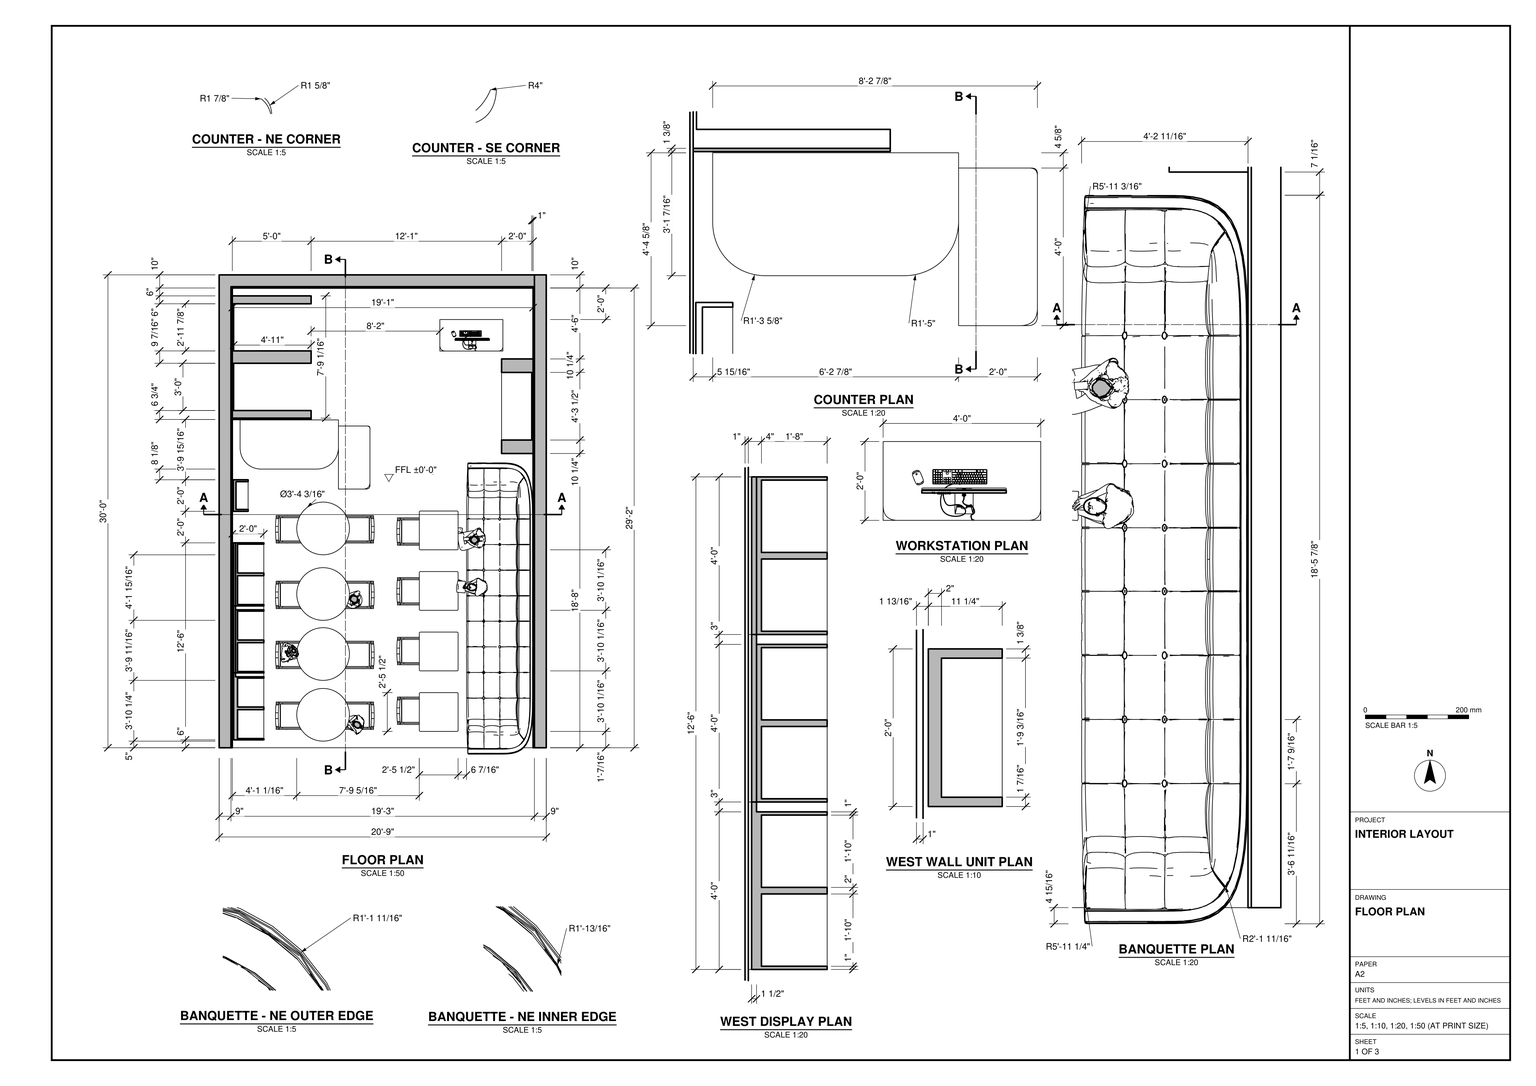
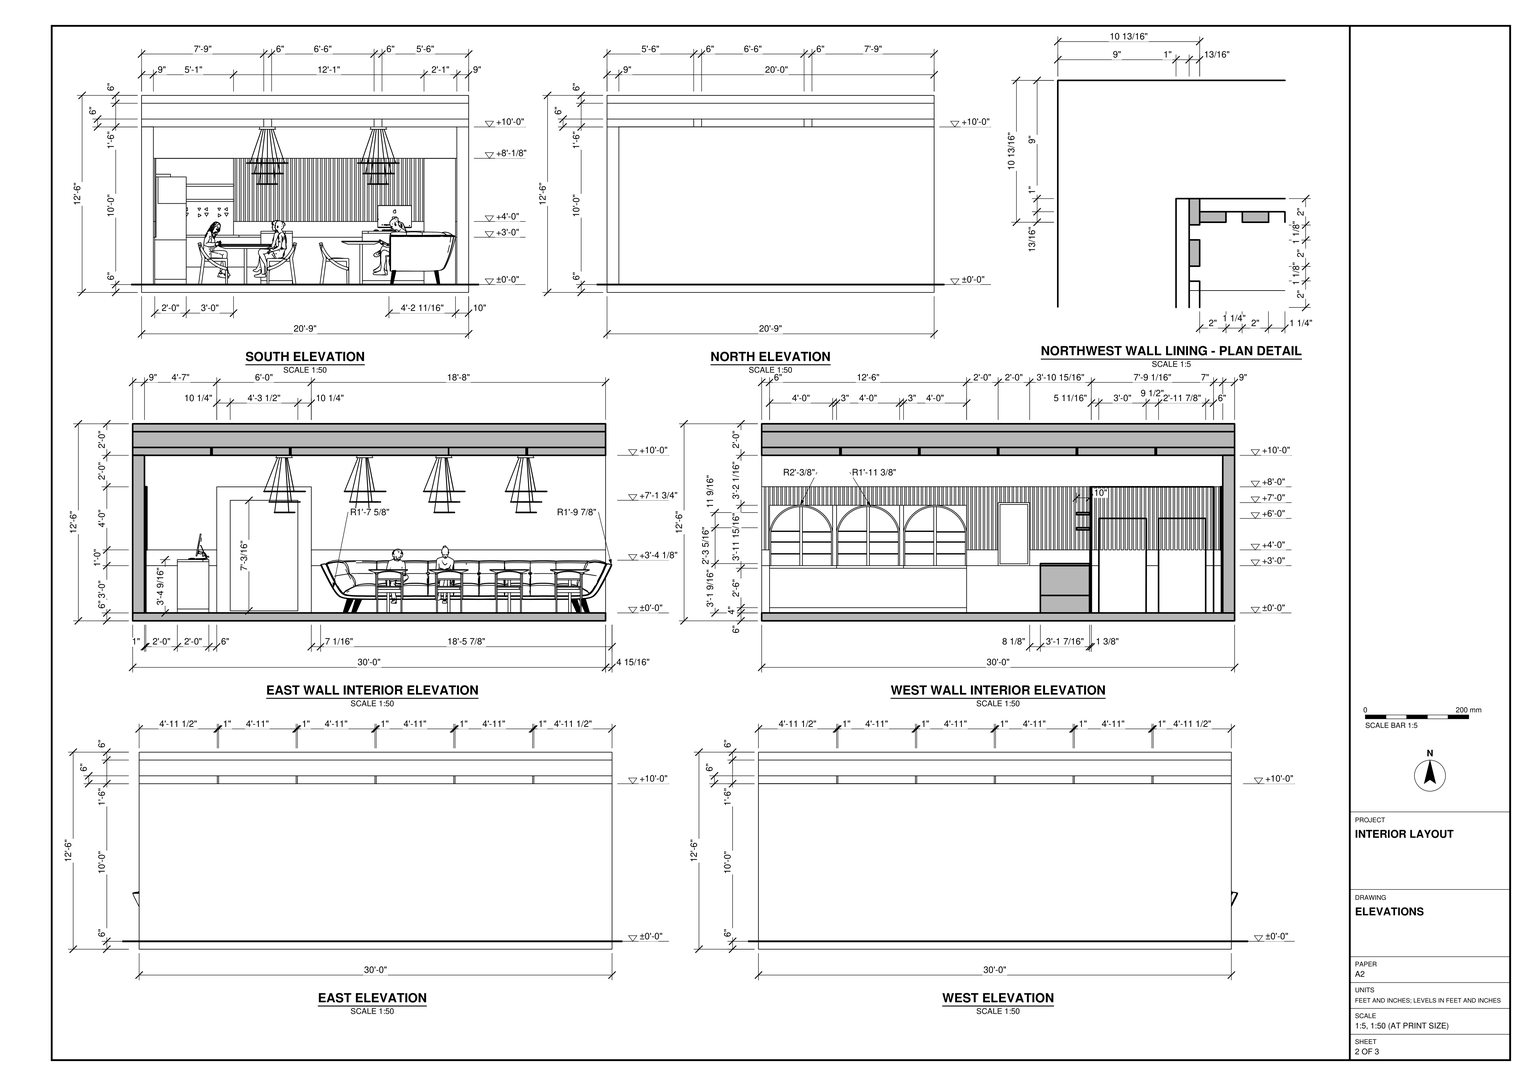
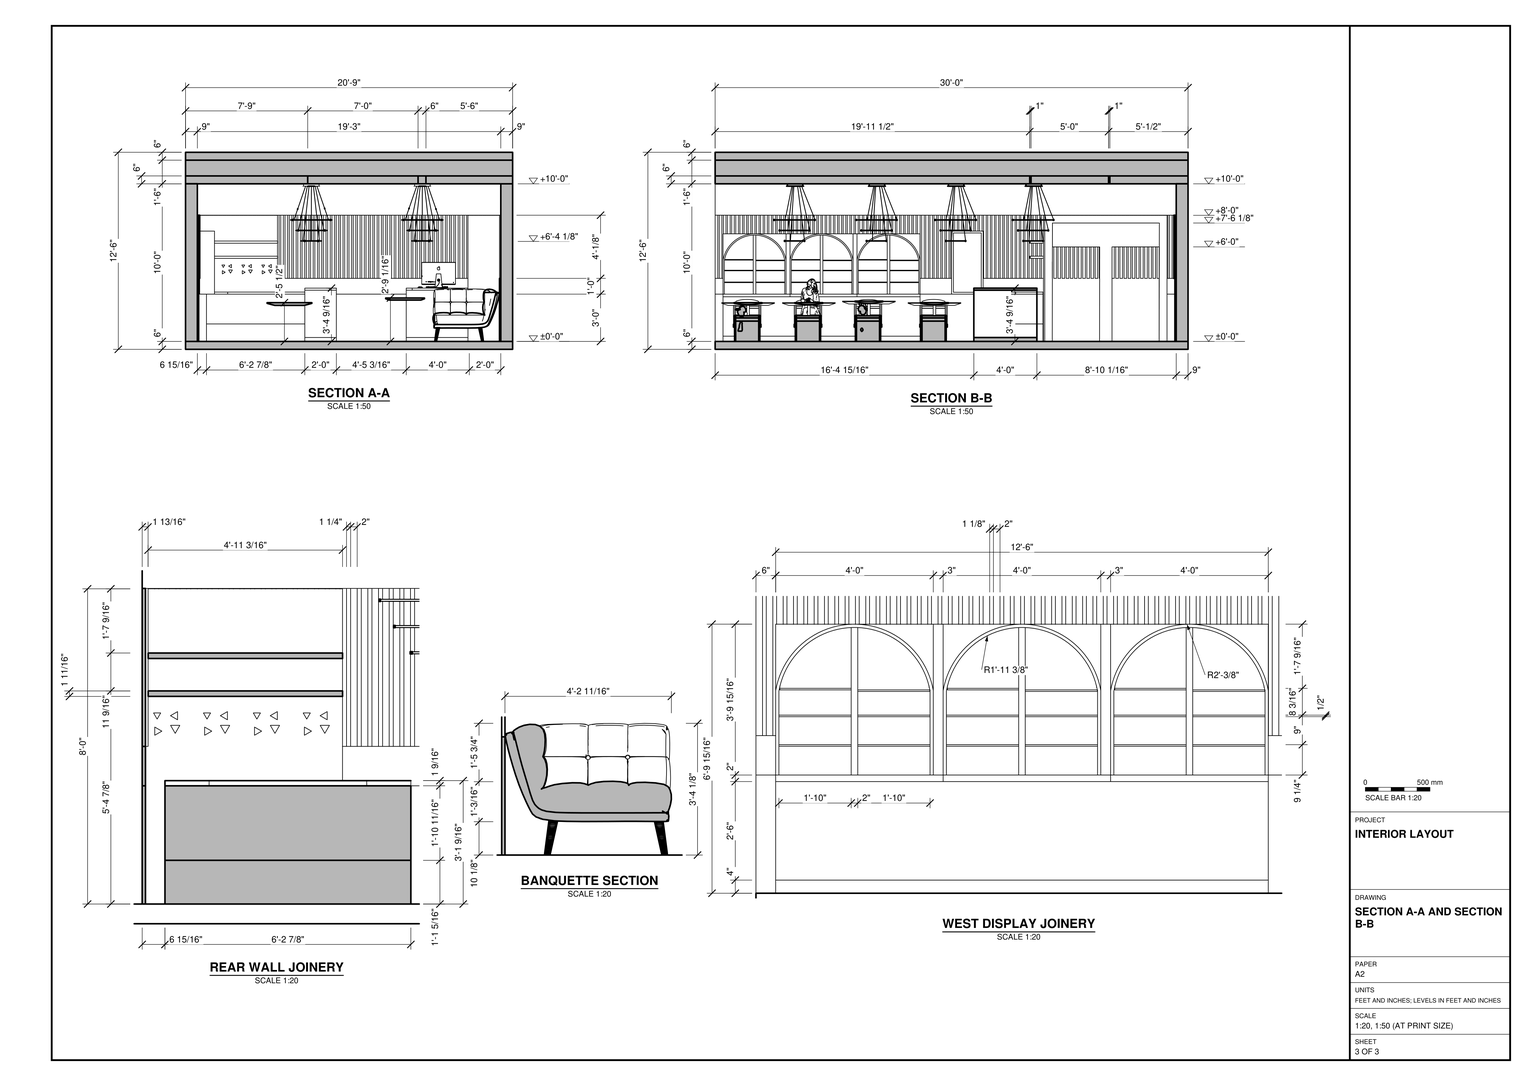
Build the single-storey café interior in SketchUp from task_files/diagram_01.pdf. Work in feet and inches. Set the finished floor at ±0'-0". The complete model measures 20'-9" east to west, 30'-4 15/16" north to south and 12'-6" in height. Use the 30'-0" shell length shown in plan rather than extending the walls to the full model length. Model the floor slab, the walls at their drawn thicknesses and the layered roof assembly. Leave the south side open beneath the overhead structure, as shown in the south elevation.

Place the long banquette against the east wall, with its curved ends and back facing the row of square tables. Arrange the round tables farther west, with chairs on opposite sides. Build the west display as three arched shelving bays on a continuous base. In the rear area, follow the details for the counter's rounded corners and projecting end, the shelves, the vertical wall lining and the framed openings. Place the separate workstation toward the northeast. Use the sections to set furniture, joinery and pendant heights relative to the finished floor.

Decor and loose items, including lights and computer equipment, may be any suitable library components. Make the shell elements and each furniture or joinery piece separate groups or components, and use components for repeated parts. Save one SketchUp model as output_files/cafe_with_banquette_seating_and_arched_display_joinery.skp.

# SketchUp Ruby script. Lengths in inches.
U = 1.inch
M = Sketchup.active_model
def pt(a) = Geom::Point3d.new(a.map { |v| v * U })
def face(e, loops, mat)
  f = e.add_face(loops[0].map { |a| pt(a) })
  loops[1..].each { |l| e.add_face(l.map { |a| pt(a) }).erase! }
  f.material = f.back_material = mat if mat
  f
end
# faces: each face lists its corners as indices into pts; further lists are holes
def faces(e, pts, list, mat = nil) = list.each { |f| face(e, (f[0].is_a?(Array) ? f : [f]).map { |l| l.map { |i| pts[i] } }, mat) }
# xy, xz, yz: faces in a plane at the given z, y or x. An outline is a flat list of corners, or four numbers for a rectangle; further outlines are holes
def ring(l) = l.size == 4 ? [[l[0], l[1]], [l[2], l[1]], [l[2], l[3]], [l[0], l[3]]] : l.each_slice(2).to_a
def flat(e, list, mat, &to3) = list.each { |f| face(e, (f[0].is_a?(Array) ? f : [f]).map { |l| ring(l).map { |u, v| to3.(u, v) } }, mat) }
def xy(e, z, list, mat = nil) = flat(e, list, mat) { |x, y| [x, y, z] }
def xz(e, y, list, mat = nil) = flat(e, list, mat) { |x, z| [x, y, z] }
def yz(e, x, list, mat = nil) = flat(e, list, mat) { |y, z| [x, y, z] }
def lines(e, pts, list) = list.each { |a, b| e.add_line(pt(pts[a]), pt(pts[b])) }
# prism: a flat outline (further loops are holes) pulled along v
def prism(e, loops, v, mat = nil)
  f = face(e, loops, mat); d = Geom::Vector3d.new(v.map { |x| x * U })
  f.pushpull(f.normal.samedirection?(d) ? d.length : -d.length)
end
def box(e, o, s, mat = nil) = prism(e, [[o, [o[0] + s[0], o[1], o[2]], [o[0] + s[0], o[1] + s[1], o[2]], [o[0], o[1] + s[1], o[2]]]], [0, 0, s[2]], mat)
def at(x, y, z, deg = 0) = Geom::Transformation.translation(pt([x, y, z])) * Geom::Transformation.rotation(ORIGIN, Z_AXIS, deg.degrees)
def axes(o, x, y, z) = Geom::Transformation.new([*x, 0, *y, 0, *z, 0, *pt(o).to_a, 1])
def part(name) = M.definitions.add(name)
# library, detail: a bought-in or finely detailed component or shape, given as its bounding box
def library(name, o, s) = part(name).tap { |d| box(d.entities, o, s) }
def detail(e, o, s) = box(e.add_group.entities, o, s)
def put(e, d, t, mat = nil) = e.add_instance(d, t).tap { |i| i.material = mat if mat }
def group(e, t, mat = nil) = e.add_group.tap { |g| g.transformation = t; g.material = mat if mat }.entities
root = M.entities
M.materials.add("0215 AP 9421 FABRIC PINK").color = [153, 66, 100]
M.materials.add("0738 AP 7691 TREE OF LIFE").color = [215, 220, 196]
M.materials.add("0754 AP 7723 SPRING BREEZE").color = [232, 231, 204]
M.materials.add("[Carrera Marble]").color = [207, 207, 207]
M.materials.add("[Color E01]").color = [255, 255, 204]
M.materials.add("[Color F01]").color = [229, 255, 204]
M.materials.add("[Color G02]").color = [153, 255, 153]
M.materials.add("[Color M01]").color = [226, 226, 226]
M.materials.add("[Color M02]").color = [198, 198, 198]
M.materials.add("d8d170801efe8ea26683d572c47f922d--composition").color = [170, 173, 176]
c1 = library("Pablo Sofa Grey",[-86,0,0],[86,35.5,29.5])
c2 = library("Component",[-22.41,-42.93,0],[44.82,85.86,134.55])
c3 = library("Component3",[-2.88,-3.29,-6.71],[5.76,6.58,13.42])
c4 = library("Component5",[-23.75,-39.51,0],[47.5,79.02,138.44])
c5 = library("Component9",[516.85,-170.02,-0.32],[47.26,71.27,113.45])
c6 = library("Square pedestal table",[0,0,0],[29.53,29.53,29.53])
c7 = library("Round pedestal table",[-5.31,-5.31,0],[40.15,40.15,29.53])
c8 = library("Liberty+Caffe+Chair",[-0.07,-0.06,0],[21.07,22.56,31.98])
c9 = library("Component7",[-3.3,-3.53,0.09],[6.88,7.63,16.11])
c10 = library("W002E06312",[-3.23,3.26,6.15],[36.28,37.2,43.85])
c11 = library("Apple iMac 27 in + keyboard + mouse",[-3.98,0.8125,-0.4],[15.55,28.93,19.63])
c12 = part("Vertical slat")
box(c12.entities,[0,0,0],[0.8,2,48.11])
c13 = library("Group\#14",[0,0,0],[24,150,47.9375])
xy(root,19.3125,[[32.08,212.15,32.22,225.58,31.99,225.59,31.77,225.6,31.35,225.66,31.16,225.71,30.98,225.76,30.8,225.83,30.64,225.9,30.49,225.98,30.34,226.08,30.21,226.18,29.97,226.42,29.87,226.55,29.69,226.85,29.62,227.01,29.55,227.1875,29.5,227.37,29.45,227.5625,29.42,227.76,29.39,227.98,29.38,228.2,29.375,228.43,29.375,249.58,77.375,249.58,77.375,228.96,77.37,228.6875,77.35,228.42,77.32,228.17,77.28,227.93,77.23,227.7,77.16,227.48,77.09,227.28,77,227.09,76.9,226.9,76.79,226.73,76.66,226.57,76.53,226.43,76.38,226.29,76.22,226.17,76.05,226.06,75.87,225.96,75.68,225.87,75.47,225.79,75.26,225.73,75.03,225.68,74.79,225.64,74.53,225.61,74.27,225.59,73.99,225.58,74.14,212.15],[32.08,212.15,31.4,212.16,31.99,225.59,32.22,225.58],[74.14,212.15,73.99,225.58,74.27,225.59,74.86,212.16],[31.4,212.16,30.55,212.22,31.77,225.6,31.99,225.59],[74.86,212.16,74.27,225.59,74.53,225.61,75.76,212.22],
  [30.55,212.22,29.65,212.32,31.56,225.63,31.77,225.6],[75.76,212.22,74.53,225.61,74.79,225.64,76.69,212.33],[29.65,212.32,28.71,212.48,31.35,225.66,31.56,225.63],[76.69,212.33,74.79,225.64,75.03,225.68,77.67,212.5],[28.71,212.48,27.73,212.71,31.16,225.71,31.35,225.66],
  [77.67,212.5,75.03,225.68,75.26,225.73,78.68,212.73],[27.73,212.71,26.72,213.01,30.98,225.76,31.16,225.71],[78.68,212.73,75.26,225.73,75.47,225.79,79.73,213.04],[26.72,213.01,25.68,213.39,30.8,225.83,30.98,225.76],[79.73,213.04,75.47,225.79,75.68,225.87,80.8,213.44],
  [25.68,213.39,24.62,213.875,30.64,225.9,30.8,225.83],[80.8,213.44,75.68,225.87,75.87,225.96,81.89,213.93],[24.62,213.875,23.56,214.45,30.49,225.98,30.64,225.9],[81.89,213.93,75.87,225.96,76.05,226.06,82.98,214.53],[23.56,214.45,22.52,215.14,30.34,226.08,30.49,225.98],
  [82.98,214.53,76.05,226.06,76.22,226.17,84.04,215.23],[22.52,215.14,21.52,215.92,30.21,226.18,30.34,226.08],[84.04,215.23,76.22,226.17,76.38,226.29,85.07,216.03],[21.52,215.92,20.58,216.79,30.09,226.3,30.21,226.18],[85.07,216.03,76.38,226.29,76.53,226.43,86.04,216.92],
  [20.58,216.79,19.71,217.73,29.97,226.42,30.09,226.3],[86.04,216.92,76.53,226.43,76.66,226.57,86.93,217.89],[19.71,217.73,18.93,218.73,29.87,226.55,29.97,226.42],[86.93,217.89,76.66,226.57,76.79,226.73,87.73,218.91],[18.93,218.73,18.25,219.77,29.78,226.7,29.87,226.55],
  [87.73,218.91,76.79,226.73,76.9,226.9,88.43,219.98],[18.25,219.77,17.67,220.83,29.69,226.85,29.78,226.7],[88.43,219.98,76.9,226.9,77,227.09,89.02,221.07],[17.67,220.83,17.1875,221.89,29.62,227.01,29.69,226.85],[89.02,221.07,77,227.09,77.09,227.28,89.52,222.15],
  [17.1875,221.89,16.8,222.93,29.55,227.1875,29.62,227.01],[89.52,222.15,77.09,227.28,77.16,227.48,89.92,223.23],[16.8,222.93,16.5,223.94,29.5,227.37,29.55,227.1875],[89.92,223.23,77.16,227.48,77.23,227.7,90.23,224.27],[16.5,223.94,16.27,224.92,29.45,227.5625,29.5,227.37],
  [90.23,224.27,77.23,227.7,77.28,227.93,90.46,225.29],[16.27,224.92,16.11,225.86,29.42,227.76,29.45,227.5625],[90.46,225.29,77.28,227.93,77.32,228.17,90.63,226.26],[16.11,225.86,16.01,226.75,29.39,227.98,29.42,227.76],[90.63,226.26,77.32,228.17,77.35,228.42,90.74,227.2],
  [16.01,226.75,15.95,227.61,29.38,228.2,29.39,227.98],[90.74,227.2,77.35,228.42,77.37,228.6875,90.8,228.1],[15.95,227.61,15.9375,228.29,29.375,228.43,29.38,228.2],[90.8,228.1,77.37,228.6875,77.375,228.96,90.8125,228.82],[15.9375,228.29,15.9375,249.58,29.375,249.58,29.375,228.43],
  [90.8125,228.82,77.375,228.96,77.375,249.58,90.8125,249.58]])
put(root,c1,axes([188.33,-4.93,6],[0,-2.57985,0],[1.4274,0,0],[0,0,1.36]))
put(root,c2,axes([190.25,122.68,13.4],[0,-0.32519,0],[0.32519,0,0],[0,0,0.32519]))
put(root,c3,axes([98.46,114.58,33.4],[-2.47299,-2.07508,0],[2.07508,-2.47299,0],[0,0,3.22826]))
put(root,c4,axes([98.06,17.49,11.55],[0,-0.31049,0],[0.31049,0,0],[0,0,0.31049]))
put(root,c5,axes([238.78,356.19,13.37],[0,-0.36517,0],[0.36517,0,0],[0,0,0.36517]))
put(root,c6,axes([152.37,41.97,6],[0,-1,0],[1,0,0],[0,0,1.12]),"d8d170801efe8ea26683d572c47f922d--composition")
put(root,c7,at(64.35,86.12,6,-90),"d8d170801efe8ea26683d572c47f922d--composition")
put(root,c8,at(65.41,60.21,6,90))
put(root,c8,axes([95.51,60.21,6],[0,1,0],[1,0,0],[0,0,1]))
put(root,c7,axes([64.35,131.82,6],[0,-1,0],[1,0,0],[0,0,1.04]),"d8d170801efe8ea26683d572c47f922d--composition")
put(root,c8,axes([95.51,105.91,6],[0,1,0],[1,0,0],[0,0,1]))
put(root,c8,at(65.41,105.91,6,90))
put(root,c7,at(64.35,181.73,6,-90),"d8d170801efe8ea26683d572c47f922d--composition")
put(root,c8,axes([95.51,155.82,6],[0,1,0],[1,0,0],[0,0,1]))
put(root,c8,at(65.41,155.82,6,90))
put(root,c7,at(64.35,39.85,6,-90),"d8d170801efe8ea26683d572c47f922d--composition")
put(root,c8,axes([95.51,13.94,6],[0,1,0],[1,0,0],[0,0,1]))
put(root,c8,at(65.41,13.94,6,90))
put(root,c9,axes([58,71.33,10.75],[0,-2.65352,0],[-2.65352,0,0],[0,0,2.65352]))
put(root,c6,axes([152.37,88.05,6],[0,-1,0],[1,0,0],[0,0,1.12]),"d8d170801efe8ea26683d572c47f922d--composition")
put(root,c6,axes([152.37,134.14,6],[0,-1,0],[1,0,0],[0,0,1.12]),"d8d170801efe8ea26683d572c47f922d--composition")
put(root,c6,axes([152.37,180.22,6],[0,-1,0],[1,0,0],[0,0,1.12]),"d8d170801efe8ea26683d572c47f922d--composition")
put(root,c8,at(157.76,17.7,6,90))
put(root,c8,at(157.76,63.18,6,90))
put(root,c8,at(157.76,108.66,6,90))
put(root,c8,at(157.76,154.14,6,90))
put(root,c10,at(80.8,41.18,76))
put(root,c10,at(80.8,103.49,76))
put(root,c10,at(80.8,163.78,76))
put(root,c10,axes([195.22,41.18,76],[-1,0,0],[0,1,0],[0,0,1]))
put(root,c10,axes([195.22,103.49,76],[-1,0,0],[0,1,0],[0,0,1]))
put(root,c10,axes([195.22,163.78,76],[-1,0,0],[0,1,0],[0,0,1]))
put(root,c10,at(80.8,222.81,76))
put(root,c10,axes([195.22,225.06,76],[-1,0,0],[0,1,0],[0,0,1]))
put(root,c11,at(206.3,305.98,46.98,90))
g1 = group(root,at(0,0,6),"[Color M02]")
prism(g1,[[[0,0,0],[0,360,0],[240,360,0],[240,351,0],[9,351,0],[9,0,0]]],[0,0,120.1])
g2 = group(root,at(240,9,6),"[Color M01]")
box(g2,[0,-9,0],[9,360,120])
g3 = group(root,at(9,0,6))
box(g3,[0,0,0],[1,351,36])
g4 = group(root,at(9,0,42))
box(g4,[0,0,0],[1,351,12])
g5 = group(root,at(9,0,54))
box(g5,[0,0,0],[1,351,48.11])
g6 = group(root,at(10,350,6))
box(g6,[0,0,0],[230,1,36])
g7 = group(root,at(10,350,42))
box(g7,[0,0,0],[230,1,12])
g8 = group(root,at(10.8,350,54))
box(g8,[0,0,0],[229.2,1,48.11])
g9 = group(root,at(10,0,54))
put(g9,c12,at(224.75,350,0,-90))
put(g9,c12,at(0,0,0))
put(g9,c12,at(215.02,350,0,-90))
put(g9,c12,at(176.07,350,0,-90))
put(g9,c12,at(169.58,350,0,-90))
put(g9,c12,at(208.53,350,0,-90))
put(g9,c12,at(166.33,350,0,-90))
put(g9,c12,at(159.84,350,0,-90))
put(g9,c12,at(218.26,350,0,-90))
put(g9,c12,at(163.09,350,0,-90))
put(g9,c12,at(179.3125,350,0,-90))
put(g9,c12,at(211.77,350,0,-90))
put(g9,c12,at(202.03,350,0,-90))
put(g9,c12,at(198.79,350,0,-90))
put(g9,c12,at(189.05,350,0,-90))
put(g9,c12,at(221.51,350,0,-90))
put(g9,c12,at(192.3,350,0,-90))
put(g9,c12,at(185.81,350,0,-90))
put(g9,c12,at(182.56,350,0,-90))
put(g9,c12,at(195.54,350,0,-90))
put(g9,c12,at(172.82,350,0,-90))
put(g9,c12,at(205.28,350,0,-90))
put(g9,c12,at(23.52,350,0,-90))
put(g9,c12,at(0.8,350,0,-90))
put(g9,c12,at(101.42,350,0,-90))
put(g9,c12,at(114.4,350,0,-90))
put(g9,c12,at(7.29,350,0,-90))
put(g9,c12,at(153.35,350,0,-90))
put(g9,c12,at(143.61,350,0,-90))
put(g9,c12,at(130.63,350,0,-90))
put(g9,c12,at(124.14,350,0,-90))
put(g9,c12,at(117.65,350,0,-90))
put(g9,c12,at(107.91,350,0,-90))
put(g9,c12,at(133.875,350,0,-90))
put(g9,c12,at(104.66,350,0,-90))
put(g9,c12,at(78.7,350,0,-90))
put(g9,c12,at(156.59,350,0,-90))
put(g9,c12,at(75.45,350,0,-90))
put(g9,c12,at(65.71,350,0,-90))
put(g9,c12,at(52.73,350,0,-90))
put(g9,c12,at(46.24,350,0,-90))
put(g9,c12,at(68.96,350,0,-90))
put(g9,c12,at(39.75,350,0,-90))
put(g9,c12,at(72.21,350,0,-90))
put(g9,c12,at(42.99,350,0,-90))
put(g9,c12,at(13.78,350,0,-90))
put(g9,c12,at(137.12,350,0,-90))
put(g9,c12,at(36.5,350,0,-90))
put(g9,c12,at(10.54,350,0,-90))
put(g9,c12,at(150.1,350,0,-90))
put(g9,c12,at(55.98,350,0,-90))
put(g9,c12,at(4.05,350,0,-90))
put(g9,c12,at(85.1875,350,0,-90))
put(g9,c12,at(140.37,350,0,-90))
put(g9,c12,at(127.38,350,0,-90))
put(g9,c12,at(20.27,350,0,-90))
put(g9,c12,at(59.22,350,0,-90))
put(g9,c12,at(120.89,350,0,-90))
put(g9,c12,at(111.15,350,0,-90))
put(g9,c12,at(81.94,350,0,-90))
put(g9,c12,at(146.86,350,0,-90))
put(g9,c12,at(94.93,350,0,-90))
put(g9,c12,at(49.49,350,0,-90))
put(g9,c12,at(30.01,350,0,-90))
put(g9,c12,at(98.17,350,0,-90))
put(g9,c12,at(26.77,350,0,-90))
put(g9,c12,at(91.68,350,0,-90))
put(g9,c12,at(33.26,350,0,-90))
put(g9,c12,at(88.43,350,0,-90))
put(g9,c12,at(17.03,350,0,-90))
put(g9,c12,at(62.47,350,0,-90))
put(g9,c12,at(0,3.14,0))
put(g9,c12,at(228,350,0,-90))
put(g9,c12,at(0,37.73,0))
put(g9,c12,at(0,6.29,0))
put(g9,c12,at(0,44.02,0))
put(g9,c12,at(0,50.31,0))
put(g9,c12,at(0,53.45,0))
put(g9,c12,at(0,56.59,0))
put(g9,c12,at(0,59.74,0))
put(g9,c12,at(0,9.43,0))
put(g9,c12,at(0,22.01,0))
put(g9,c12,at(0,12.58,0))
put(g9,c12,at(0,25.15,0))
put(g9,c12,at(0,47.16,0))
put(g9,c12,at(0,28.3,0))
put(g9,c12,at(0,15.72,0))
put(g9,c12,at(0,18.86,0))
put(g9,c12,at(0,31.44,0))
put(g9,c12,at(0,34.59,0))
put(g9,c12,at(0,40.875,0))
put(g9,c12,at(0,254.68,0))
put(g9,c12,at(0,106.9,0))
put(g9,c12,at(0,147.77,0))
put(g9,c12,at(0,172.93,0))
put(g9,c12,at(0,113.1875,0))
put(g9,c12,at(0,144.63,0))
put(g9,c12,at(0,138.34,0))
put(g9,c12,at(0,91.18,0))
put(g9,c12,at(0,100.61,0))
put(g9,c12,at(0,160.35,0))
put(g9,c12,at(0,188.65,0))
put(g9,c12,at(0,81.75,0))
put(g9,c12,at(0,116.33,0))
put(g9,c12,at(0,103.76,0))
put(g9,c12,at(0,75.46,0))
put(g9,c12,at(0,201.23,0))
put(g9,c12,at(0,210.66,0))
put(g9,c12,at(0,213.8,0))
put(g9,c12,at(0,110.05,0))
put(g9,c12,at(0,150.92,0))
put(g9,c12,at(0,216.95,0))
put(g9,c12,at(0,238.95,0))
put(g9,c12,at(0,163.5,0))
put(g9,c12,at(0,245.24,0))
put(g9,c12,at(0,94.32,0))
put(g9,c12,at(0,72.32,0))
put(g9,c12,at(0,176.07,0))
put(g9,c12,at(0,97.47,0))
put(g9,c12,at(0,191.79,0))
put(g9,c12,at(0,119.48,0))
put(g9,c12,at(0,242.1,0))
put(g9,c12,at(0,132.05,0))
put(g9,c12,at(0,185.5,0))
put(g9,c12,at(0,122.62,0))
put(g9,c12,at(0,84.89,0))
put(g9,c12,at(0,204.37,0))
put(g9,c12,at(0,207.51,0))
put(g9,c12,at(0,179.22,0))
put(g9,c12,at(0,248.39,0))
put(g9,c12,at(0,78.6,0))
put(g9,c12,at(0,125.77,0))
put(g9,c12,at(0,88.04,0))
put(g9,c12,at(0,141.49,0))
put(g9,c12,at(0,154.0625,0))
put(g9,c12,at(0,169.78,0))
put(g9,c12,at(0,182.36,0))
put(g9,c12,at(0,223.23,0))
put(g9,c12,at(0,198.08,0))
put(g9,c12,at(0,232.67,0))
put(g9,c12,at(0,166.64,0))
put(g9,c12,at(0,69.17,0))
put(g9,c12,at(0,62.88,0))
put(g9,c12,at(0,135.2,0))
put(g9,c12,at(0,194.9375,0))
put(g9,c12,at(0,226.38,0))
put(g9,c12,at(0,66.03,0))
put(g9,c12,at(0,157.21,0))
put(g9,c12,at(0,220.09,0))
put(g9,c12,at(0,235.8125,0))
put(g9,c12,at(0,251.53,0))
put(g9,c12,at(0,128.91,0))
put(g9,c12,at(0,257.82,0))
put(g9,c12,at(0,260.96,0))
put(g9,c12,at(0,229.52,0))
put(g9,c12,at(0,342.71,0))
put(g9,c12,at(0,330.14,0))
put(g9,c12,at(0,336.42,0))
put(g9,c12,at(0,333.28,0))
put(g9,c12,at(0,289.26,0))
put(g9,c12,at(0,270.4,0))
put(g9,c12,at(0,279.83,0))
put(g9,c12,at(0,267.25,0))
put(g9,c12,at(0,264.11,0))
put(g9,c12,at(0,314.41,0))
put(g9,c12,at(0,282.97,0))
put(g9,c12,at(0,273.54,0))
put(g9,c12,at(0,320.7,0))
put(g9,c12,at(0,286.12,0))
put(g9,c12,at(0,323.85,0))
put(g9,c12,at(0,311.27,0))
put(g9,c12,at(0,345.86,0))
put(g9,c12,at(0,304.98,0))
put(g9,c12,at(0,276.68,0))
put(g9,c12,at(0,349,0))
put(g9,c12,at(0,339.57,0))
put(g9,c12,at(0,295.55,0))
put(g9,c12,at(0,298.69,0))
put(g9,c12,at(0,292.41,0))
put(g9,c12,at(0,317.56,0))
put(g9,c12,at(0,301.84,0))
put(g9,c12,at(0,308.125,0))
put(g9,c12,at(0,326.99,0))
g10 = group(root,at(10,6,6),"[Color F01]")
box(g10,[0,0,0],[24,150,4])
g11 = group(root,at(10,6,10),"[Color E01]")
box(g11,[0,0,0],[24,150,30])
put(root,c13,at(10,6,40),"[Color G02]")
g12 = group(root,at(10.8,180,42),"0215 AP 9421 FABRIC PINK")
xy(g12,0,[[0,0,11.25,24]])
xy(g12,1.41,[[2,1.41,11.25,22.59]])
xy(g12,46.59,[[2,1.41,11.25,22.59]])
xy(g12,48,[[0,0,11.25,24]])
xz(g12,0,[[0,0,11.25,48]])
xz(g12,1.41,[[2,1.41,11.25,46.59]])
xz(g12,22.59,[[2,1.41,11.25,46.59]])
xz(g12,24,[[0,0,11.25,48]])
yz(g12,0,[[0,0,24,48]])
yz(g12,2,[[1.41,1.41,22.59,46.59]])
yz(g12,11.25,[[[0,0,24,48],[1.41,1.41,22.59,46.59]]])
g13 = group(root,at(29.375,225.58,6),"0738 AP 7691 TREE OF LIFE")
xy(g13,0,[[2.71,-13.4375,2.85,0,2.62,0,2.39,0.02,2.18,0.04,1.98,0.08,1.79,0.125,1.6,0.18,1.43,0.24,1.11,0.4,0.97,0.49,0.71,0.71,0.49,0.97,0.4,1.11,0.24,1.43,0.18,1.6,0.125,1.79,0.08,1.98,0.04,2.18,0.02,2.39,0,2.62,0,24,48,24,48,3.38,47.99,3.1,47.98,2.84,47.95,2.59,47.91,2.35,47.85,2.12,47.79,1.9,47.71,1.7,47.625,1.5,47.52,1.32,47.41,1.15,47.29,0.99,47.01,0.71,46.85,0.59,46.68,0.48,46.5,0.375,46.3,0.29,46.1,0.21,45.88,0.15,45.65,0.09,45.41,0.05,45.16,0.02,44.9,0.01,44.62,0,44.76,-13.4375],[2.71,-13.4375,2.03,-13.42,2.62,0,2.85,0],[44.76,-13.4375,44.62,0,44.9,0.01,45.49,-13.42],[2.03,-13.42,1.17,-13.37,2.39,0.02,2.62,0],[45.49,-13.42,44.9,0.01,45.16,0.02,46.38,-13.36],
  [1.17,-13.37,0.27,-13.26,2.18,0.04,2.39,0.02],[46.38,-13.36,45.16,0.02,45.41,0.05,47.32,-13.25],[0.27,-13.26,-0.66,-13.1,1.98,0.08,2.18,0.04],[47.32,-13.25,45.41,0.05,45.65,0.09,48.3,-13.09],[-0.66,-13.1,-1.64,-12.875,1.79,0.125,1.98,0.08],
  [48.3,-13.09,45.65,0.09,45.88,0.15,49.31,-12.85],[-1.64,-12.875,-2.66,-12.57,1.6,0.18,1.79,0.125],[49.31,-12.85,45.88,0.15,46.1,0.21,50.36,-12.54],[-2.66,-12.57,-3.7,-12.1875,1.43,0.24,1.6,0.18],[50.36,-12.54,46.1,0.21,46.3,0.29,51.43,-12.14],
  [-3.7,-12.1875,-4.75,-11.71,1.27,0.32,1.43,0.24],[51.43,-12.14,46.3,0.29,46.5,0.375,52.52,-11.65],[-4.75,-11.71,-5.81,-11.13,1.11,0.4,1.27,0.32],[52.52,-11.65,46.5,0.375,46.68,0.48,53.6,-11.05],[-5.81,-11.13,-6.85,-10.45,0.97,0.49,1.11,0.4],
  [53.6,-11.05,46.68,0.48,46.85,0.59,54.67,-10.35],[-6.85,-10.45,-7.85,-9.67,0.84,0.6,0.97,0.49],[54.67,-10.35,46.85,0.59,47.01,0.71,55.7,-9.56],[-7.85,-9.67,-8.8,-8.8,0.71,0.71,0.84,0.6],[55.7,-9.56,47.01,0.71,47.15,0.85,56.66,-8.66],
  [-8.8,-8.8,-9.67,-7.85,0.6,0.84,0.71,0.71],[56.66,-8.66,47.15,0.85,47.29,0.99,57.56,-7.7],[-9.67,-7.85,-10.45,-6.85,0.49,0.97,0.6,0.84],[57.56,-7.7,47.29,0.99,47.41,1.15,58.35,-6.67],[-10.45,-6.85,-11.13,-5.81,0.4,1.11,0.49,0.97],
  [58.35,-6.67,47.41,1.15,47.52,1.32,59.05,-5.6],[-11.13,-5.81,-11.71,-4.75,0.32,1.27,0.4,1.11],[59.05,-5.6,47.52,1.32,47.625,1.5,59.65,-4.52],[-11.71,-4.75,-12.1875,-3.7,0.24,1.43,0.32,1.27],[59.65,-4.52,47.625,1.5,47.71,1.7,60.14,-3.43],
  [-12.1875,-3.7,-12.57,-2.66,0.18,1.6,0.24,1.43],[60.14,-3.43,47.71,1.7,47.79,1.9,60.54,-2.36],[-12.57,-2.66,-12.875,-1.64,0.125,1.79,0.18,1.6],[60.54,-2.36,47.79,1.9,47.85,2.12,60.85,-1.31],[-12.875,-1.64,-13.1,-0.66,0.08,1.98,0.125,1.79],
  [60.85,-1.31,47.85,2.12,47.91,2.35,61.09,-0.3],[-13.1,-0.66,-13.26,0.27,0.04,2.18,0.08,1.98],[61.09,-0.3,47.91,2.35,47.95,2.59,61.25,0.68],[-13.26,0.27,-13.37,1.17,0.02,2.39,0.04,2.18],[61.25,0.68,47.95,2.59,47.98,2.84,61.36,1.62],
  [-13.37,1.17,-13.42,2.03,0,2.62,0.02,2.39],[61.36,1.62,47.98,2.84,47.99,3.1,61.42,2.51],[-13.42,2.03,-13.4375,2.71,0,2.85,0,2.62],[61.42,2.51,47.99,3.1,48,3.38,61.4375,3.24],[-13.4375,2.71,-13.4375,24,0,24,0,2.85],
  [61.4375,3.24,48,3.38,48,24,61.4375,24]])
xy(g13,36,[[2.71,-13.4375,44.76,-13.4375,45.49,-13.42,46.38,-13.36,47.32,-13.25,48.3,-13.09,49.31,-12.85,50.36,-12.54,51.43,-12.14,52.52,-11.65,53.6,-11.05,54.67,-10.35,55.7,-9.56,56.66,-8.66,57.56,-7.7,58.35,-6.67,59.05,-5.6,59.65,-4.52,60.14,-3.43,60.54,-2.36,60.85,-1.31,61.09,-0.3,61.25,0.68,61.36,1.62,61.42,2.51,61.4375,3.24,61.4375,24,-13.4375,24,-13.4375,2.71,-13.42,2.03,-13.37,1.17,-13.26,0.27,-13.1,-0.66,-12.875,-1.64,-12.57,-2.66,-12.1875,-3.7,-11.71,-4.75,-11.13,-5.81,-10.45,-6.85,-9.67,-7.85,-8.8,-8.8,-7.85,-9.67,-6.85,-10.45,-5.81,-11.13,-4.75,-11.71,-3.7,-12.1875,-2.66,-12.57,-1.64,-12.875,-0.66,-13.1,0.27,-13.26,1.17,-13.37,2.03,-13.42]])
xz(g13,-13.4375,[[2.71,0,44.76,36]])
xz(g13,24,[[-13.4375,0,0,36],[0,0,48,36],[48,0,61.4375,36]])
yz(g13,-13.4375,[[2.71,0,24,36]])
yz(g13,61.4375,[[3.24,0,24,36]])
p = [[1.17,-13.37,0],[1.17,-13.37,36],[0.27,-13.26,36],[0.27,-13.26,0],[2.03,-13.42,0],[2.03,-13.42,36],
  [2.71,-13.4375,0],[2.71,-13.4375,36],[44.76,-13.4375,0],[45.49,-13.42,0],[45.49,-13.42,36],[44.76,-13.4375,36],
  [46.38,-13.36,0],[46.38,-13.36,36],[47.32,-13.25,0],[47.32,-13.25,36],[-0.66,-13.1,36],[-0.66,-13.1,0],
  [48.3,-13.09,0],[48.3,-13.09,36],[-1.64,-12.875,36],[-1.64,-12.875,0],[49.31,-12.85,0],[49.31,-12.85,36],
  [-2.66,-12.57,36],[-2.66,-12.57,0],[50.36,-12.54,0],[50.36,-12.54,36],[-3.7,-12.1875,36],[-3.7,-12.1875,0],
  [51.43,-12.14,0],[51.43,-12.14,36],[-4.75,-11.71,36],[-4.75,-11.71,0],[52.52,-11.65,0],[52.52,-11.65,36],
  [-5.81,-11.13,36],[-5.81,-11.13,0],[53.6,-11.05,0],[53.6,-11.05,36],[-6.85,-10.45,36],[-6.85,-10.45,0],
  [54.67,-10.35,0],[54.67,-10.35,36],[-7.85,-9.67,36],[-7.85,-9.67,0],[55.7,-9.56,0],[55.7,-9.56,36],
  [-8.8,-8.8,36],[-8.8,-8.8,0],[56.66,-8.66,0],[56.66,-8.66,36],[-9.67,-7.85,36],[-9.67,-7.85,0],
  [57.56,-7.7,0],[57.56,-7.7,36],[-10.45,-6.85,36],[-10.45,-6.85,0],[58.35,-6.67,0],[58.35,-6.67,36],
  [-11.13,-5.81,36],[-11.13,-5.81,0],[59.05,-5.6,0],[59.05,-5.6,36],[-11.71,-4.75,36],[-11.71,-4.75,0],
  [59.65,-4.52,0],[59.65,-4.52,36],[-12.1875,-3.7,36],[-12.1875,-3.7,0],[60.14,-3.43,0],[60.14,-3.43,36],
  [-12.57,-2.66,36],[-12.57,-2.66,0],[60.54,-2.36,0],[60.54,-2.36,36],[-12.875,-1.64,36],[-12.875,-1.64,0],
  [60.85,-1.31,0],[60.85,-1.31,36],[-13.1,-0.66,36],[-13.1,-0.66,0],[61.09,-0.3,0],[61.09,-0.3,36],
  [-13.26,0.27,36],[-13.26,0.27,0],[61.25,0.68,0],[61.25,0.68,36],[-13.37,1.17,36],[-13.37,1.17,0],
  [61.36,1.62,0],[61.36,1.62,36],[-13.42,2.03,36],[-13.42,2.03,0],[61.42,2.51,0],[61.42,2.51,36],
  [-13.4375,2.71,36],[-13.4375,2.71,0],[61.4375,3.24,0],[61.4375,3.24,36]]
faces(g13,p,[[0,1,2,3],[0,4,5,1],[6,7,5,4],[8,9,10,11],[12,13,10,9],[14,15,13,12],[3,2,16,17],[18,19,15,14],
  [17,16,20,21],[22,23,19,18],[21,20,24,25],[26,27,23,22],[25,24,28,29],[30,31,27,26],[29,28,32,33],[34,35,31,30],
  [33,32,36,37],[38,39,35,34],[37,36,40,41],[42,43,39,38],[41,40,44,45],[46,47,43,42],[45,44,48,49],[50,51,47,46],
  [48,52,53,49],[50,54,55,51],[52,56,57,53],[54,58,59,55],[56,60,61,57],[58,62,63,59],[60,64,65,61],[62,66,67,63],
  [64,68,69,65],[66,70,71,67],[68,72,73,69],[70,74,75,71],[72,76,77,73],[74,78,79,75],[76,80,81,77],[78,82,83,79],
  [80,84,85,81],[82,86,87,83],[84,88,89,85],[86,90,91,87],[88,92,93,89],[90,94,95,91],[92,96,97,93],[94,98,99,95]])
g14 = group(root,at(90.8125,244.9375,6,-90))
prism(g14,[[[45.03,24,0],[45.27,23.99,0],[45.5,23.98,0],[45.72,23.95,0],[45.94,23.92,0],[46.14,23.87,0],[46.33,23.8125,0],[46.51,23.75,0],[46.68,23.67,0],[46.84,23.58,0],[46.99,23.48,0],[47.13,23.375,0],[47.26,23.26,0],[47.375,23.13,0],[47.48,22.99,0],[47.58,22.84,0],[47.67,22.68,0],[47.75,22.51,0],[47.8125,22.33,0],[47.87,22.14,0],[47.92,21.94,0],[47.95,21.72,0],[47.98,21.5,0],[47.99,21.27,0],[48,21.03,0],[48,0,0],[0,0,0],[0,22.22,0],[0,22.36,0],[0.01,22.5,0],[0.03,22.63,0],[0.05,22.76,0],[0.08,22.88,0],[0.11,23,0],[0.15,23.1,0],[0.2,23.21,0],[0.25,23.3,0],[0.31,23.39,0],[0.375,23.48,0],[0.45,23.55,0],[0.52,23.625,0],[0.61,23.69,0],[0.7,23.75,0],[0.79,23.8,0],[0.9,23.85,0],[1,23.89,0],[1.12,23.92,0],[1.24,23.95,0],[1.37,23.97,0],[1.5,23.99,0],[1.64,24,0],[1.78,24,0]]],[0,0,3])
g15 = group(root,at(90.8125,244.9375,9,-90),"0738 AP 7691 TREE OF LIFE")
prism(g15,[[[42.62,24,0],[43.06,23.99,0],[43.48,23.96,0],[43.88,23.92,0],[44.26,23.85,0],[44.625,23.77,0],[44.97,23.66,0],[45.3,23.54,0],[45.61,23.4,0],[45.9,23.24,0],[46.17,23.07,0],[46.42,22.87,0],[46.65,22.65,0],[46.87,22.42,0],[47.07,22.17,0],[47.24,21.9,0],[47.4,21.61,0],[47.54,21.3,0],[47.66,20.97,0],[47.77,20.625,0],[47.85,20.26,0],[47.92,19.88,0],[47.96,19.48,0],[47.99,19.06,0],[48,18.62,0],[48,0,0],[0,0,0],[0,21.62,0],[0,21.8125,0],[0.02,22,0],[0.04,22.18,0],[0.07,22.35,0],[0.1,22.51,0],[0.15,22.66,0],[0.2,22.8,0],[0.26,22.94,0],[0.33,23.07,0],[0.41,23.1875,0],[0.5,23.3,0],[0.6,23.4,0],[0.7,23.5,0],[0.8125,23.59,0],[0.93,23.67,0],[1.06,23.74,0],[1.2,23.8,0],[1.34,23.85,0],[1.49,23.9,0],[1.65,23.93,0],[1.82,23.96,0],[2,23.98,0],[2.1875,24,0],[2.38,24,0]]],[0,0,36])
g16 = group(root,at(10,250.9375,6),"0215 AP 9421 FABRIC PINK")
xy(g16,72,[[1,51.1875,60,87.0625]])
xy(g16,96,[[0,0,60,93.0625]])
xz(g16,0,[[0,0,60,96]])
xz(g16,51.1875,[[1,0,60,72]])
xz(g16,87.0625,[[1,0,60,72]])
xz(g16,93.0625,[[0,0,60,96]])
yz(g16,0,[[0,0,93.0625,96]])
yz(g16,1,[[41.69,0,41.8125,71.9375,5.8125,72,5.69,0.0625],[51.1875,0,87.0625,72]])
yz(g16,60,[[0,0,5.69,0,5.69,0.0625,5.8125,72,5.85,90.15,87.22,90.15,87.0625,0,93.0625,0,93.0625,96,0,96],[41.69,0,51.1875,0,51.1875,72,87.0625,72,87.0625,0,87.22,90.15,5.85,90.15,5.8125,72,41.8125,71.9375]])
p = [[60,41.69,0],[60,41.8125,71.9375],[1,41.8125,71.9375],[1,41.69,0],[60,5.8125,72],[60,5.69,0.0625],
  [1,5.69,0.0625],[1,5.8125,72]]
faces(g16,p,[[0,1,2,3],[4,5,6,7],[1,4,7,2]])
g17 = group(root,at(10.8,239.39,80.77))
prism(g17,[[[0,10,0],[59.2,10.55,0],[59.29,0.55,0],[0.09,0,0]]],[0,0,1.67])
g18 = group(root,at(10.8,239.39,69.23))
prism(g18,[[[0,10,0],[59.2,10.55,0],[59.29,0.55,0],[0.09,0,0]]],[0,0,1.67])
g19 = group(root,at(10,249.9375,6),"0215 AP 9421 FABRIC PINK")
prism(g19,[[[60,1,0],[0,1,0],[0,1,96],[60,1,96]],[[9.05,1,51.98],[10.46,1,54.41],[7.64,1,54.41]],[[24.24,1,51.98],[25.65,1,54.41],[22.83,1,54.41]],[[39.43,1,51.98],[40.83,1,54.41],[38.02,1,54.41]],[[54.61,1,51.98],[56.02,1,54.41],[53.21,1,54.41]],[[2.83,1,51.4],[4.99,1,52.65],[2.83,1,53.89]],[[18.02,1,51.4],[20.17,1,52.65],[18.02,1,53.89]],[[33.2,1,51.4],[35.36,1,52.65],[33.2,1,53.89]],[[48.39,1,51.4],[50.55,1,52.65],[48.39,1,53.89]],[[9.77,1,58.6],[7.61,1,57.35],[9.77,1,56.11]],[[24.96,1,58.6],[22.8,1,57.35],[24.96,1,56.11]],[[40.14,1,58.6],[37.99,1,57.35],[40.14,1,56.11]],[[55.33,1,58.6],[53.18,1,57.35],[55.33,1,56.11]],[[2.47,1,58.19],[3.55,1,56.32],[4.63,1,58.19]],[[17.65,1,58.19],[18.74,1,56.32],[19.82,1,58.19]],[[32.84,1,58.19],[33.92,1,56.32],[35.01,1,58.19]],[[48.03,1,58.19],[49.11,1,56.32],[50.19,1,58.19]]],[0,-1,0])
g20 = group(root,at(168,302,6),"0754 AP 7723 SPRING BREEZE")
box(g20,[0,0,0],[48,24,3])
g21 = group(root,at(168,302,9),"0738 AP 7691 TREE OF LIFE")
prism(g21,[[[48,24,0],[48,3.77,0],[47.99,3.46,0],[47.97,3.17,0],[47.94,2.88,0],[47.9,2.62,0],[47.84,2.36,0],[47.76,2.12,0],[47.68,1.89,0],[47.58,1.67,0],[47.47,1.47,0],[47.35,1.28,0],[47.21,1.11,0],[47.06,0.94,0],[46.89,0.79,0],[46.72,0.65,0],[46.53,0.53,0],[46.33,0.42,0],[46.11,0.32,0],[45.88,0.24,0],[45.64,0.16,0],[45.38,0.1,0],[45.12,0.06,0],[44.83,0.03,0],[44.54,0.01,0],[44.23,0,0],[4.53,0,0],[4.16,0.01,0],[3.8,0.03,0],[3.47,0.07,0],[3.14,0.125,0],[2.84,0.2,0],[2.55,0.28,0],[2.27,0.39,0],[2.01,0.5,0],[1.77,0.64,0],[1.54,0.79,0],[1.33,0.95,0],[1.13,1.13,0],[0.95,1.33,0],[0.79,1.54,0],[0.64,1.77,0],[0.5,2.01,0],[0.39,2.27,0],[0.28,2.55,0],[0.2,2.84,0],[0.125,3.14,0],[0.07,3.47,0],[0.03,3.8,0],[0.01,4.16,0],[0,4.53,0],[0,24,0]]],[0,0,36])
g22 = group(root,at(168,302,45),"0754 AP 7723 SPRING BREEZE")
prism(g22,[[[44.54,0.01,0],[44.23,0,0],[4.53,0,0],[4.16,0.01,0],[3.8,0.03,0],[3.47,0.07,0],[3.14,0.125,0],[2.84,0.2,0],[2.55,0.28,0],[2.27,0.39,0],[2.01,0.5,0],[1.77,0.64,0],[1.54,0.79,0],[1.33,0.95,0],[1.13,1.13,0],[0.95,1.33,0],[0.79,1.54,0],[0.64,1.77,0],[0.5,2.01,0],[0.39,2.27,0],[0.28,2.55,0],[0.2,2.84,0],[0.125,3.14,0],[0.07,3.47,0],[0.03,3.8,0],[0.01,4.16,0],[0,4.53,0],[0,24,0],[48,24,0],[48,3.77,0],[47.99,3.46,0],[47.97,3.17,0],[47.94,2.88,0],[47.9,2.62,0],[47.84,2.36,0],[47.76,2.12,0],[47.68,1.89,0],[47.58,1.67,0],[47.47,1.47,0],[47.35,1.28,0],[47.21,1.11,0],[47.06,0.94,0],[46.89,0.79,0],[46.72,0.65,0],[46.53,0.53,0],[46.33,0.42,0],[46.11,0.32,0],[45.88,0.24,0],[45.64,0.16,0],[45.38,0.1,0],[45.12,0.06,0],[44.83,0.03,0]]],[0,0,1.57])
g23 = group(root,at(215,224,6),"0215 AP 9421 FABRIC PINK")
xy(g23,0,[[0,0,24,72]])
xy(g23,1.57,[[0,10.25,23,61.73]])
xy(g23,85.74,[[0,10.26,23,61.74]])
xy(g23,96,[[0,0,24,72]])
xz(g23,0,[[0,0,24,96]])
xz(g23,72,[[0,0,24,96]])
yz(g23,0,[[[0,0,72,96],[10.25,1.57,61.73,1.57,61.74,85.74,10.26,85.74]]])
yz(g23,23,[[10.25,1.57,10.26,85.74,61.74,85.74,61.73,1.57]])
yz(g23,24,[[0,0,72,96]])
p = [[0,10.25,1.57],[0,10.26,85.74],[23,10.26,85.74],[23,10.25,1.57],[0,61.74,85.74],[0,61.73,1.57],
  [23,61.73,1.57],[23,61.74,85.74]]
faces(g23,p,[[0,1,2,3],[4,5,6,7]])
g24 = group(root,at(239,0,42))
box(g24,[0,0,0],[1,350,12])
g25 = group(root,at(239,0,30))
box(g25,[0,0,-24],[1,350,36])
g26 = group(root,at(0,0,126),"[Color M01]")
box(g26,[0,0,0],[249,360,6])
g27 = group(root,at(90.8125,196.9375,45),"0754 AP 7723 SPRING BREEZE")
prism(g27,[[[18.62,0,0],[0,0,0],[0,48,0],[21.62,48,0],[21.8125,48,0],[22,47.98,0],[22.18,47.96,0],[22.35,47.93,0],[22.51,47.9,0],[22.66,47.85,0],[22.8,47.8,0],[22.94,47.74,0],[23.07,47.67,0],[23.1875,47.59,0],[23.3,47.5,0],[23.4,47.4,0],[23.5,47.3,0],[23.59,47.1875,0],[23.67,47.07,0],[23.74,46.94,0],[23.8,46.8,0],[23.85,46.66,0],[23.9,46.51,0],[23.93,46.35,0],[23.96,46.18,0],[23.98,46,0],[24,45.8125,0],[24,45.62,0],[24,5.38,0],[23.99,4.94,0],[23.96,4.52,0],[23.92,4.12,0],[23.85,3.74,0],[23.77,3.375,0],[23.66,3.03,0],[23.54,2.7,0],[23.4,2.39,0],[23.24,2.1,0],[23.07,1.83,0],[22.87,1.58,0],[22.65,1.35,0],[22.42,1.13,0],[22.17,0.93,0],[21.9,0.76,0],[21.61,0.6,0],[21.3,0.46,0],[20.97,0.34,0],[20.625,0.23,0],[20.26,0.15,0],[19.88,0.08,0],[19.48,0.04,0],[19.06,0.01,0]]],[0,0,1.57])
g28 = group(root,at(15.9375,201.58,42),"0754 AP 7723 SPRING BREEZE")
xy(g28,1.57,[[16.14,10.5625,58.2,10.5625,58.92,10.58,59.82,10.64,60.76,10.75,61.73,10.91,62.75,11.15,63.79,11.46,64.87,11.86,65.95,12.35,67.04,12.95,68.11,13.65,69.13,14.44,70.1,15.34,70.99,16.3,71.79,17.33,72.49,18.4,73.09,19.48,73.58,20.57,73.98,21.64,74.29,22.69,74.52,23.7,74.69,24.68,74.8,25.62,74.86,26.51,74.875,27.24,74.875,48,0,48,0,26.71,0.01,26.03,0.07,25.17,0.18,24.27,0.34,23.34,0.5625,22.36,0.86,21.34,1.25,20.3,1.73,19.25,2.31,18.19,2.99,17.15,3.77,16.15,4.64,15.2,5.58,14.33,6.59,13.55,7.63,12.87,8.68,12.29,9.74,11.8125,10.78,11.43,11.79,11.125,12.77,10.9,13.71,10.74,14.61,10.63,15.46,10.58]])
xz(g28,10.5625,[[16.14,0,58.2,1.57]])
xz(g28,48,[[0,0,13.4375,1.57],[13.4375,0,61.4375,1.57],[61.4375,0,74.875,1.57]])
yz(g28,0,[[26.71,0,48,1.57]])
p = [[13.71,10.74,0],[14.61,10.63,0],[14.61,10.63,1.57],[13.71,10.74,1.57],[15.46,10.58,0],[15.46,10.58,1.57],
  [16.14,10.5625,0],[16.14,10.5625,1.57],[58.2,10.5625,0],[58.92,10.58,0],[58.92,10.58,1.57],[58.2,10.5625,1.57],
  [59.82,10.64,0],[59.82,10.64,1.57],[60.76,10.75,0],[60.76,10.75,1.57],[12.77,10.9,0],[12.77,10.9,1.57],
  [61.73,10.91,0],[61.73,10.91,1.57],[11.79,11.125,0],[11.79,11.125,1.57],[62.75,11.15,0],[62.75,11.15,1.57],
  [10.78,11.43,0],[10.78,11.43,1.57],[63.79,11.46,0],[63.79,11.46,1.57],[9.74,11.8125,0],[9.74,11.8125,1.57],
  [64.87,11.86,0],[64.87,11.86,1.57],[8.68,12.29,0],[8.68,12.29,1.57],[65.95,12.35,0],[65.95,12.35,1.57],
  [7.63,12.87,0],[7.63,12.87,1.57],[67.04,12.95,0],[67.04,12.95,1.57],[6.59,13.55,0],[6.59,13.55,1.57],
  [68.11,13.65,0],[68.11,13.65,1.57],[5.58,14.33,0],[5.58,14.33,1.57],[69.13,14.44,0],[69.13,14.44,1.57],
  [4.64,15.2,0],[4.64,15.2,1.57],[70.1,15.34,0],[70.1,15.34,1.57],[3.77,16.15,0],[3.77,16.15,1.57],
  [70.99,16.3,0],[70.99,16.3,1.57],[2.99,17.15,0],[2.99,17.15,1.57],[71.79,17.33,0],[71.79,17.33,1.57],
  [2.31,18.19,0],[2.31,18.19,1.57],[72.49,18.4,0],[72.49,18.4,1.57],[1.73,19.25,0],[1.73,19.25,1.57],
  [73.09,19.48,0],[73.09,19.48,1.57],[1.25,20.3,0],[1.25,20.3,1.57],[73.58,20.57,0],[73.58,20.57,1.57],
  [0.86,21.34,0],[0.86,21.34,1.57],[73.98,21.64,0],[73.98,21.64,1.57],[0.5625,22.36,0],[0.5625,22.36,1.57],
  [74.29,22.69,0],[74.29,22.69,1.57],[0.34,23.34,0],[0.34,23.34,1.57],[74.52,23.7,0],[74.52,23.7,1.57],
  [0.18,24.27,0],[0.18,24.27,1.57],[74.69,24.68,0],[74.69,24.68,1.57],[0.07,25.17,0],[0.07,25.17,1.57],
  [74.8,25.62,0],[74.8,25.62,1.57],[0.01,26.03,0],[0.01,26.03,1.57],[74.86,26.51,0],[74.86,26.51,1.57],
  [0,26.71,0],[0,26.71,1.57],[74.875,27.24,0],[74.875,27.24,1.57]]
faces(g28,p,[[0,1,2,3],[1,4,5,2],[4,6,7,5],[8,9,10,11],[9,12,13,10],[12,14,15,13],[16,0,3,17],[14,18,19,15],
  [20,16,17,21],[18,22,23,19],[24,20,21,25],[22,26,27,23],[28,24,25,29],[26,30,31,27],[32,28,29,33],[30,34,35,31],
  [36,32,33,37],[34,38,39,35],[40,36,37,41],[38,42,43,39],[44,40,41,45],[42,46,47,43],[48,44,45,49],[46,50,51,47],
  [52,48,49,53],[50,54,55,51],[56,52,53,57],[54,58,59,55],[60,56,57,61],[58,62,63,59],[64,60,61,65],[62,66,67,63],
  [68,64,65,69],[66,70,71,67],[72,68,69,73],[70,74,75,71],[76,72,73,77],[74,78,79,75],[80,76,77,81],[78,82,83,79],
  [84,80,81,85],[82,86,87,83],[88,84,85,89],[86,90,91,87],[92,88,89,93],[90,94,95,91],[96,92,93,97],[94,98,99,95]])
g29 = group(root,at(0,0,0),"[Carrera Marble]")
box(g29,[0,0,0],[249,360,6])
g30 = group(root,at(0,0,144))
box(g30,[0,0,0],[249,360,6])
g31 = group(root,at(0,0,126))
xy(g31,0,[[0,0,93,59.5],[99,0,177.01,59.5],[183.01,0,249,59.5],[0,60.5,93,119.5],[99,60.5,177.01,119.5],
  [183.01,60.5,249,119.5],[0,120.5,93,179.5],[99,120.5,177.01,179.5],[183.01,120.5,249,179.5],[0,180.5,93,239.5],
  [99,180.5,177.01,239.5],[183.01,180.5,249,239.5],[96,239.5,180,240.5],[0,240.5,93,299.5],[99,240.5,177.01,299.5],
  [183.01,240.5,249,299.5],[96,299.5,180,300.5],[0,300.5,93,360],[99,300.5,177.01,360],[183.01,300.5,249,360]])
xy(g31,6,[[93,0,93,59.5,0,59.5,0,60.5,93,60.5,93,119.5,0,119.5,0,120.5,93,120.5,93,179.5,0,179.5,0,180.5,93,180.5,93,239.5,99,239.5,99,180.5,249,180.5,249,179.5,99,179.5,99,120.5,249,120.5,249,119.5,99,119.5,99,60.5,177.01,60.5,177.01,59.5,99,59.5,99,0],[177.01,0,183.01,59.5],[177.01,59.5,180,60.5],[180,59.5,249,60.5],[177.01,60.5,183.01,119.5],
  [177.01,120.5,183.01,179.5],[177.01,180.5,183.01,239.5],[0,239.5,249,240.5],[93,240.5,99,299.5],[177.01,240.5,183.01,299.5],
  [0,299.5,249,300.5],[93,300.5,99,360],[177.01,300.5,183.01,360]])
xy(g31,18,[[0,0,249,360]])
xz(g31,0,[[0,0,93,0,93,6,99,6,99,0,177.01,0,177.01,6,183.01,6,183.01,0,249,0,249,18,0,18]])
xz(g31,59.5,[[0,0,93,6],[99,0,177.01,6],[183.01,0,249,6]])
xz(g31,60.5,[[0,0,93,6],[99,0,177.01,6],[183.01,0,249,6]])
xz(g31,119.5,[[0,0,93,6],[99,0,177.01,6],[177.01,0,180,6],[183.01,0,249,6]])
xz(g31,120.5,[[0,0,93,6],[177.01,0,180,6],[183.01,0,249,6]])
xz(g31,179.5,[[0,0,93,6],[177.01,0,180,6],[183.01,0,249,6]])
xz(g31,180.5,[[0,0,93,6],[177.01,0,180,6],[183.01,0,249,6]])
xz(g31,239.5,[[0,0,93,6],[96,0,99,6],[99,0,177.01,6],[177.01,0,180,6],[183.01,0,249,6]])
xz(g31,240.5,[[0,0,93,6],[96,0,99,6],[99,0,177.01,6],[177.01,0,180,6],[183.01,0,249,6]])
xz(g31,299.5,[[0,0,93,6],[96,0,99,6],[99,0,177.01,6],[177.01,0,180,6],[183.01,0,249,6]])
xz(g31,300.5,[[0,0,93,6],[96,0,99,6],[99,0,177.01,6],[177.01,0,180,6],[183.01,0,249,6]])
xz(g31,360,[[0,0,0,18,249,18,249,0,183.01,0,183.01,6,177.01,6,177.01,0,99,0,99,6,93,6,93,0]])
yz(g31,0,[[0,0,0,18,360,18,360,0,300.5,0,300.5,6,299.5,6,299.5,0,240.5,0,240.5,6,239.5,6,239.5,0,180.5,0,180.5,6,179.5,6,179.5,0,120.5,0,120.5,6,119.5,6,119.5,0,60.5,0,60.5,6,59.5,6,59.5,0]])
yz(g31,93,[[0,0,59.5,6],[60.5,0,119.5,6],[120.5,0,179.5,6],[180.5,0,239.5,6],[240.5,0,299.5,6],
  [300.5,0,360,6]])
yz(g31,99,[[0,0,59.5,6],[60.5,0,119.5,6],[240.5,0,299.5,6],[300.5,0,360,6]])
yz(g31,177.01,[[0,0,59.5,6],[59.5,0,60.5,6],[60.5,0,119.5,6],[120.5,0,179.5,6],[180.5,0,239.5,6],
  [240.5,0,299.5,6],[300.5,0,360,6]])
yz(g31,180,[[59.5,0,60.5,6]])
yz(g31,183.01,[[0,0,59.5,6],[60.5,0,119.5,6],[120.5,0,179.5,6],[180.5,0,239.5,6],[240.5,0,299.5,6],
  [300.5,0,360,6]])
yz(g31,249,[[0,0,59.5,0,59.5,6,60.5,6,60.5,0,119.5,0,119.5,6,120.5,6,120.5,0,179.5,0,179.5,6,180.5,6,180.5,0,239.5,0,239.5,6,240.5,6,240.5,0,299.5,0,299.5,6,300.5,6,300.5,0,360,0,360,18,0,18]])
p = [[96,59.5,0],[96,60.5,0],[96,119.5,0],[96,120.5,0],[96,179.5,0],[96,180.5,0],
  [180,179.5,0],[180,180.5,0],[180,119.5,0],[180,120.5,0],[96,179.5,6],[99,179.5,6],
  [99,179.5,0]]
lines(g31,p,[[0,1],[2,3],[4,5],[6,7],[8,9],[10,11],[4,12],[4,10]])
